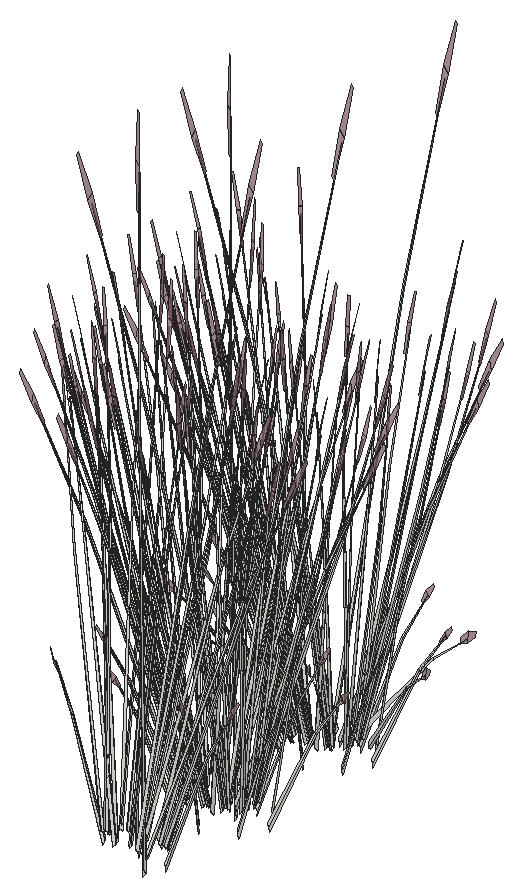
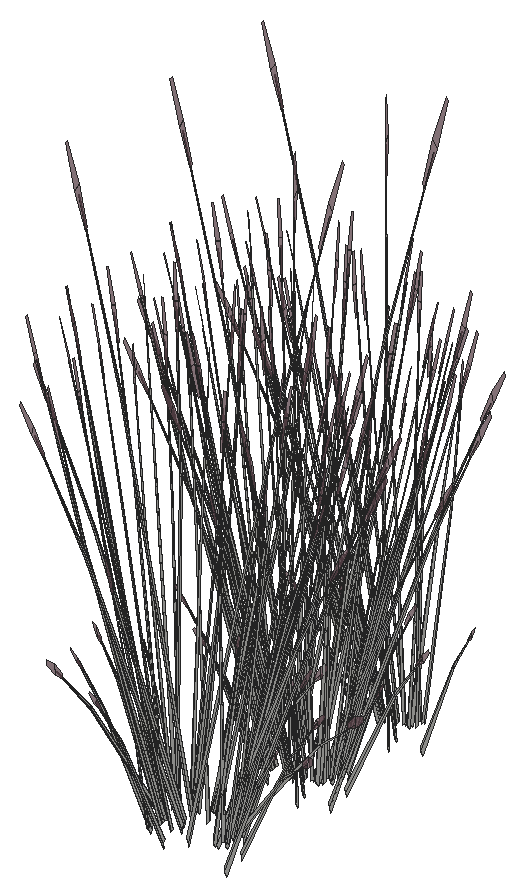
# SketchUp Ruby script. Lengths in inches.
U = 1.inch
M = Sketchup.active_model
def pt(a) = Geom::Point3d.new(a.map { |v| v * U })
def face(e, loops, mat)
  f = e.add_face(loops[0].map { |a| pt(a) })
  loops[1..].each { |l| e.add_face(l.map { |a| pt(a) }).erase! }
  f.material = f.back_material = mat if mat
  f
end
# faces: each face lists its corners as indices into pts; further lists are holes
def faces(e, pts, list, mat = nil) = list.each { |f| face(e, (f[0].is_a?(Array) ? f : [f]).map { |l| l.map { |i| pts[i] } }, mat) }
# xy, xz, yz: faces in a plane at the given z, y or x. An outline is a flat list of corners, or four numbers for a rectangle; further outlines are holes
def ring(l) = l.size == 4 ? [[l[0], l[1]], [l[2], l[1]], [l[2], l[3]], [l[0], l[3]]] : l.each_slice(2).to_a
def flat(e, list, mat, &to3) = list.each { |f| face(e, (f[0].is_a?(Array) ? f : [f]).map { |l| ring(l).map { |u, v| to3.(u, v) } }, mat) }
def xy(e, z, list, mat = nil) = flat(e, list, mat) { |x, y| [x, y, z] }
def xz(e, y, list, mat = nil) = flat(e, list, mat) { |x, z| [x, y, z] }
def yz(e, x, list, mat = nil) = flat(e, list, mat) { |y, z| [x, y, z] }
def lines(e, pts, list) = list.each { |a, b| e.add_line(pt(pts[a]), pt(pts[b])) }
# prism: a flat outline (further loops are holes) pulled along v
def prism(e, loops, v, mat = nil)
  f = face(e, loops, mat); d = Geom::Vector3d.new(v.map { |x| x * U })
  f.pushpull(f.normal.samedirection?(d) ? d.length : -d.length)
end
def box(e, o, s, mat = nil) = prism(e, [[o, [o[0] + s[0], o[1], o[2]], [o[0] + s[0], o[1] + s[1], o[2]], [o[0], o[1] + s[1], o[2]]]], [0, 0, s[2]], mat)
def at(x, y, z, deg = 0) = Geom::Transformation.translation(pt([x, y, z])) * Geom::Transformation.rotation(ORIGIN, Z_AXIS, deg.degrees)
def axes(o, x, y, z) = Geom::Transformation.new([*x, 0, *y, 0, *z, 0, *pt(o).to_a, 1])
def part(name) = M.definitions.add(name)
# library, detail: a bought-in or finely detailed component or shape, given as its bounding box
def library(name, o, s) = part(name).tap { |d| box(d.entities, o, s) }
def detail(e, o, s) = box(e.add_group.entities, o, s)
def put(e, d, t, mat = nil) = e.add_instance(d, t).tap { |i| i.material = mat if mat }
def group(e, t, mat = nil) = e.add_group.tap { |g| g.transformation = t; g.material = mat if mat }.entities
root = M.entities
M.materials.add("LightPink_Translucent").color = [144, 107, 117]
M.materials["LightPink_Translucent"].alpha = 0.75
c1 = part("blade")
p = [[2.15,0.21,22],[0,0.17,0],[0.09,0.45,0],[2.18,0.31,22],[2.29,0.31,22],[0.38,0.45,0],
  [2.48,0.24,33],[2.49,0.24,33],[2.48,0.22,33]]
faces(c1.entities,p,[[0,1,2,3],[4,5,2,3],[6,3,4,7],[8,0,3,6]])
c2 = part("seeds")
p = [[0.3,-0.1,1.38],[-0.01,-0.03,1.59],[-0.01,-0.03,0.03],[0.14,-0.07,-0.07],[0.29,-0.03,3],[0.15,0.01,3.11]]
faces(c2.entities,p,[[0,1,2,3],[1,0,4,5]],"LightPink_Translucent")
c3 = part("blade with seeds")
put(c3.entities,c1,at(0,0,0))
put(c3.entities,c2,axes([2.4,0.25,30.99],[1.5799,-0.05474,1.17369],[-0.12525,1.92788,0.29478],[-0.07173,-0.02425,1.56792]))
put(root,c3,axes([335.46,443.875,52.4],[0.50473,0.00941,-0.62776],[-0.0339,0.39618,0.07576],[0.21383,0.04181,0.88802]))
put(root,c3,axes([330.7,444.37,50.44],[0.21042,-0.1771,1.01491],[0.08303,0.28036,0.74569],[-0.15207,0.0502,0.22354]))
put(root,c3,axes([335.77,444.04,52],[0.28729,0.24465,-0.31292],[-0.32804,0.23159,0.40398],[0.16667,0.03524,0.77298]))
put(root,c3,axes([331.49,443.6,52],[-0.43951,0.05584,-0.31292],[-0.11606,-0.31924,0.40398],[-0.12595,0.08575,0.77298]))
put(root,c3,axes([334.73,443.41,51.43],[-0.18755,-0.06732,1.51428],[0.38813,-0.28243,0.12244],[0.24191,0.12741,0.64734]))
put(root,c3,axes([334.77,442.53,51.95],[-0.4363,-0.20303,1.22187],[0.46069,-0.31611,0.5272],[0.14077,0.1905,1.18105]))
put(root,c3,axes([331.625,443.38,52.45],[0.46706,0.21546,-0.10745],[-0.26908,0.31203,-0.59638],[-0.13196,0.10846,0.90619]))
put(root,c3,axes([335.43,444.18,50.44],[-0.28429,-0.11236,1.01491],[0.36709,-0.11416,0.74569],[0.09901,0.0967,0.22354]))
put(root,c3,axes([334.43,444.5,52.45],[0.30087,-0.33447,-0.10745],[0.43572,0.19269,-0.59638],[0.15146,0.0945,0.90619]))
put(root,c3,axes([332.25,443.29,51.43],[0.12611,-0.12006,1.51428],[0.31843,0.32408,0.12244],[-0.2184,0.14759,0.64734]))
put(root,c3,axes([331.86,443.64,52.14],[0.12971,0.3568,-0.45151],[-0.49122,0.06241,-0.34973],[-0.14077,0.09583,0.86392]))
put(root,c3,axes([334.74,442.91,50.51],[-0.01379,-0.36791,1.24828],[0.62424,0.09537,0.52853],[-0.14764,0.20132,1.17828]))
put(root,c3,axes([334.79,444.33,52.14],[0.49824,-0.09289,-0.45151],[0.08716,0.35177,-0.34973],[0.13382,0.10081,0.86392]))
put(root,c3,axes([332.69,449.72,51.43],[0.11542,0.12546,1.51428],[-0.53333,0.10562,0.12244],[-0.12054,-0.19696,0.64734]))
put(root,c3,axes([334.11,449.8125,52.4],[-0.24099,-0.31773,-0.62776],[0.49607,-0.17707,0.07576],[-0.05635,-0.15352,0.88802]))
put(root,c3,axes([332.16,443.58,51.43],[0.09401,-0.13431,1.51428],[0.3944,0.27795,0.12244],[-0.17792,0.17323,0.64734]))
put(root,c3,axes([332.27,444.34,52],[-0.34164,0.20573,-0.31292],[-0.3234,-0.23491,0.40398],[-0.04921,0.11936,0.77298]))
put(root,c3,axes([333.25,444.51,52.45],[0.49409,-0.18193,-0.10745],[0.24281,0.32289,-0.59638],[0.06519,0.13607,0.90619]))
put(root,c3,axes([335.12,450.125,52.4],[0.01314,-0.36145,-0.62776],[0.55324,0.02428,0.07576],[0.05838,-0.15313,0.88802]))
put(root,c3,axes([332.48,445.14,50.44],[-0.01307,-0.23234,1.01491],[0.32652,0.16572,0.74569],[-0.06422,0.11074,0.22354]))
put(root,c3,axes([334.16,449.54,52],[0.15222,-0.30049,-0.31292],[0.44409,0.08764,0.40398],[-0.04072,-0.12098,0.77298]))
put(root,c3,axes([334.5,449.94,51.43],[-0.09401,0.13431,1.51428],[-0.3944,-0.27795,0.12244],[0.17792,-0.17323,0.64734]))
put(root,c3,axes([332.61,444.24,52.42],[0.36145,0.26255,-0.50118],[-0.38183,0.22994,-0.3882],[-0.055,0.1334,0.95895]))
put(root,c3,axes([333.93,449.75,52.14],[-0.49634,-0.09796,-0.45151],[0.17013,-0.33585,-0.34973],[-0.04551,-0.13522,0.86392]))
put(root,c3,axes([334.24,448.91,50.44],[0.06477,0.22786,1.01491],[-0.35932,-0.1262,0.74569],[0.03867,-0.11667,0.22354]))
put(root,c3,axes([333.68,444.5,52.14],[0.49634,0.09796,-0.45151],[-0.17013,0.33585,-0.34973],[0.04551,0.13522,0.86392]))
put(root,c3,axes([335.01,450,52.14],[-0.36145,-0.26255,-0.45151],[0.38183,-0.22994,-0.34973],[0.055,-0.1334,0.86392]))
put(root,c3,axes([333.96,443.8,51.43],[-0.11542,-0.12546,1.51428],[0.53333,-0.10562,0.12244],[0.12054,0.19696,0.64734]))
put(root,c3,axes([333.45,444.7,52],[-0.15222,0.30049,-0.31292],[-0.44409,-0.08764,0.40398],[0.04072,0.12098,0.77298]))
put(root,c3,axes([332.49,444.12,52.72],[-0.01314,0.36145,-0.69681],[-0.55324,-0.02428,0.08409],[-0.05838,0.15313,0.9857]))
put(root,c3,axes([334.36,449.73,52.45],[-0.49409,0.18193,-0.10745],[-0.24281,-0.32289,-0.59638],[-0.06519,-0.13607,0.90619]))
put(root,c3,axes([335.38,450.14,52.45],[-0.55492,-0.01936,-0.10745],[0.01517,-0.36657,-0.59638],[0.03855,-0.14118,0.90619]))
put(root,c3,axes([335.35,449.91,52],[0.34164,-0.20573,-0.31292],[0.3234,0.23491,0.40398],[0.04921,-0.11936,0.77298]))
put(root,c3,axes([332.39,449.18,50.44],[0.26338,0.136,1.01491],[-0.38358,0.08175,0.74569],[-0.08207,-0.10452,0.22354]))
put(root,c3,axes([333.03,449.9,52.4],[-0.43054,-0.18887,-0.62776],[0.30598,-0.33097,0.07576],[-0.15599,-0.11277,0.88802]))
put(root,c3,axes([333.02,443.87,51.43],[-0.01236,-0.14998,1.51428],[0.53562,0.09949,0.12244],[-0.03313,0.21373,0.64734]))
put(root,c3,axes([332.88,449.65,52],[-0.07798,-0.31474,-0.31292],[0.44579,-0.08311,0.40398],[-0.11974,-0.09019,0.77298]))
put(root,c3,axes([333.5,444.43,52.4],[0.24099,0.31773,-0.62776],[-0.49607,0.17707,0.07576],[0.05635,0.15352,0.88802]))
put(root,c3,axes([331.92,450.11,51.43],[0.18755,0.06732,1.51428],[-0.38813,0.28243,0.12244],[-0.24191,-0.12741,0.64734]))
put(root,c3,axes([332.83,449.91,52.14],[-0.49824,0.09289,-0.45151],[-0.08716,-0.35177,-0.34973],[-0.13382,-0.10081,0.86392]))
put(root,c3,axes([332.31,444.63,50.97],[0.01109,-0.20172,1.3638],[0.49896,0.10655,0.18846],[-0.04323,0.21498,0.64398]))
put(root,c3,axes([335.77,450.75,52.4],[0.26374,-0.30832,-0.62776],[0.46217,0.21911,0.07576],[0.15748,-0.11171,0.88802]))
put(root,c3,axes([335.76,450.61,52.14],[-0.12971,-0.3568,-0.45151],[0.49122,-0.06241,-0.34973],[0.14077,-0.09583,0.86392]))
put(root,c3,axes([335.99,450.86,52.45],[-0.46706,-0.21546,-0.10745],[0.26908,-0.31203,-0.59638],[0.13196,-0.10846,0.90619]))
put(root,c3,axes([334.06,452.04,50.9375],[0.43633,0.15757,1.33654],[-0.42745,0.33945,0.52853],[-0.19146,-0.20119,1.12046]))
put(root,c3,axes([336.36,449.9,50.44],[-0.16818,0.19891,1.01491],[-0.14456,-0.26725,0.74569],[0.1389,-0.06697,0.22354]))
put(root,c3,axes([336.12,450.65,52],[0.43951,-0.05584,-0.31292],[0.11606,0.31924,0.40398],[0.12595,-0.08575,0.77298]))
put(root,c3,axes([331.85,450.21,52],[-0.28729,-0.24465,-0.31292],[0.32804,-0.23159,0.40398],[-0.16667,-0.03524,0.77298]))
put(root,c3,axes([332.15,450.37,52.4],[-0.50473,-0.00941,-0.62776],[0.0339,-0.39618,0.07576],[-0.21383,-0.04181,0.88802]))
put(root,c3,axes([331.98,450.45,52.14],[-0.36663,0.25884,-0.45151],[-0.32109,-0.27343,-0.34973],[-0.18628,-0.03938,0.86392]))
put(root,c3,axes([331.16,450.79,50.44],[0.32236,-0.02796,1.01491],[-0.20448,0.24636,0.74569],[-0.1593,-0.03696,0.22354]))
put(root,c3,axes([332.18,450.18,52.45],[-0.02704,0.39739,-0.10745],[-0.51189,-0.01086,-0.59638],[-0.19715,-0.0276,0.90619]))
put(root,c3,axes([336.01,451.7,52.45],[-0.25405,-0.35383,-0.10745],[0.45089,-0.17388,-0.59638],[0.19001,-0.04668,0.90619]))
put(root,c3,axes([335.98,451.4,52.14],[0.13679,-0.35544,-0.45151],[0.46898,0.12183,-0.34973],[0.18882,-0.03259,0.86392]))
put(root,c3,axes([331.52,450.73,51.43],[0.20943,-0.00885,1.51428],[-0.13893,0.38357,0.12244],[-0.29846,-0.02372,0.64734]))
put(root,c3,axes([335.9,451.53,52.4],[0.44368,-0.17257,-0.62776],[0.24726,0.35524,0.07576],[0.21437,-0.04035,0.88802]))
put(root,c3,axes([336.27,451.5625,52],[0.41962,0.10901,-0.31292],[-0.12239,0.31802,0.40398],[0.16894,-0.02916,0.77298]))
put(root,c3,axes([331.34,451.06,52],[-0.41962,-0.10901,-0.31292],[0.12239,-0.31802,0.40398],[-0.16894,0.02916,0.77298]))
put(root,c3,axes([335.13,451.17,51.43],[-0.20943,0.00885,1.51428],[0.13893,-0.38357,0.12244],[0.29846,0.02372,0.64734]))
put(root,c3,axes([332.62,451,50.95],[0.14352,-0.05653,1.56454],[0.04949,0.39467,0.12244],[-0.31087,0.05237,0.55918]))
put(root,c3,axes([337.16,451.63,50.44],[-0.31197,0.06451,1.01491],[0.14684,-0.26661,0.74569],[0.1655,0.01824,0.22354]))
put(root,c3,axes([331.63,451.22,52.14],[-0.13679,0.35544,-0.45151],[-0.46898,-0.12183,-0.34973],[-0.18882,0.03259,0.86392]))
put(root,c3,axes([331.61,450.91,52.45],[0.25405,0.35383,-0.10745],[-0.45089,0.17388,-0.59638],[-0.19001,0.04668,0.90619]))
put(root,c3,axes([336.62,452.45,51.47],[-0.09664,-0.32847,-0.03085],[0.45676,-0.07551,-0.13989],[0.09538,0.02082,0.4614]))
put(root,c3,axes([335.4375,452.44,52.45],[0.02704,-0.39739,-0.10745],[0.51189,0.01086,-0.59638],[0.19715,0.0276,0.90619]))
put(root,c3,axes([331.61,451.4,51.43],[0.17519,-0.08265,1.51428],[0.14749,0.38193,0.12244],[-0.27504,0.08632,0.64734]))
put(root,c3,axes([335.46,452.25,52.4],[0.50473,0.00941,-0.62776],[-0.0339,0.39618,0.07576],[0.21383,0.04181,0.88802]))
put(root,c3,axes([330.7,452.74,50.44],[0.21042,-0.1771,1.01491],[0.08303,0.28036,0.74569],[-0.15207,0.0502,0.22354]))
put(root,c3,axes([335.77,452.41,52],[0.28729,0.24465,-0.31292],[-0.32804,0.23159,0.40398],[0.16667,0.03524,0.77298]))
put(root,c3,axes([331.49,451.97,52],[-0.43951,0.05584,-0.31292],[-0.11606,-0.31924,0.40398],[-0.12595,0.08575,0.77298]))
put(root,c3,axes([334.73,451.79,51.43],[-0.18755,-0.06732,1.51428],[0.38813,-0.28243,0.12244],[0.24191,0.12741,0.64734]))
put(root,c3,axes([334.77,450.9,51.95],[-0.4363,-0.20303,1.22187],[0.46069,-0.31611,0.5272],[0.14077,0.1905,1.18105]))
put(root,c3,axes([331.625,451.76,52.45],[0.46706,0.21546,-0.10745],[-0.26908,0.31203,-0.59638],[-0.13196,0.10846,0.90619]))
put(root,c3,axes([335.43,452.55,50.44],[-0.28429,-0.11236,1.01491],[0.36709,-0.11416,0.74569],[0.09901,0.0967,0.22354]))
put(root,c3,axes([334.43,452.87,52.45],[0.30087,-0.33447,-0.10745],[0.43572,0.19269,-0.59638],[0.15146,0.0945,0.90619]))
put(root,c3,axes([332.25,451.66,51.43],[0.12611,-0.12006,1.51428],[0.31843,0.32408,0.12244],[-0.2184,0.14759,0.64734]))
put(root,c3,axes([331.86,452.01,52.14],[0.12971,0.3568,-0.45151],[-0.49122,0.06241,-0.34973],[-0.14077,0.09583,0.86392]))
put(root,c3,axes([334.74,451.29,50.51],[-0.01379,-0.36791,1.24828],[0.62424,0.09537,0.52853],[-0.14764,0.20132,1.17828]))
put(root,c3,axes([334.79,452.71,52.14],[0.49824,-0.09289,-0.45151],[0.08716,0.35177,-0.34973],[0.13382,0.10081,0.86392]))
put(root,c3,axes([332.16,451.96,51.43],[0.09401,-0.13431,1.51428],[0.3944,0.27795,0.12244],[-0.17792,0.17323,0.64734]))
put(root,c3,axes([332.27,452.71,52],[-0.34164,0.20573,-0.31292],[-0.3234,-0.23491,0.40398],[-0.04921,0.11936,0.77298]))
put(root,c3,axes([333.25,452.89,52.45],[0.49409,-0.18193,-0.10745],[0.24281,0.32289,-0.59638],[0.06519,0.13607,0.90619]))
put(root,c3,axes([332.48,453.51,50.44],[-0.01307,-0.23234,1.01491],[0.32652,0.16572,0.74569],[-0.06422,0.11074,0.22354]))
put(root,c3,axes([332.61,452.62,52.42],[0.36145,0.26255,-0.50118],[-0.38183,0.22994,-0.3882],[-0.055,0.1334,0.95895]))
put(root,c3,axes([333.68,452.87,52.14],[0.49634,0.09796,-0.45151],[-0.17013,0.33585,-0.34973],[0.04551,0.13522,0.86392]))
put(root,c3,axes([333.96,452.18,51.43],[-0.11542,-0.12546,1.51428],[0.53333,-0.10562,0.12244],[0.12054,0.19696,0.64734]))
put(root,c3,axes([333.45,453.08,52],[-0.15222,0.30049,-0.31292],[-0.44409,-0.08764,0.40398],[0.04072,0.12098,0.77298]))
put(root,c3,axes([332.49,452.5,52.72],[-0.01314,0.36145,-0.69681],[-0.55324,-0.02428,0.08409],[-0.05838,0.15313,0.9857]))
put(root,c3,axes([332.69,459.23,51.43],[0.11542,0.12546,1.51428],[-0.53333,0.10562,0.12244],[-0.12054,-0.19696,0.64734]))
put(root,c3,axes([333.02,452.24,51.43],[-0.01236,-0.14998,1.51428],[0.53562,0.09949,0.12244],[-0.03313,0.21373,0.64734]))
put(root,c3,axes([333.57,458.4,52.17],[-0.07723,-0.05479,1.54581],[-0.51538,0.03473,-0.24447],[-0.08225,-0.13104,0.12397]))
put(root,c3,axes([334.11,459.33,52.4],[-0.24099,-0.31773,-0.62776],[0.49607,-0.17707,0.07576],[-0.05635,-0.15352,0.88802]))
put(root,c3,axes([333.5,452.81,52.4],[0.24099,0.31773,-0.62776],[-0.49607,0.17707,0.07576],[0.05635,0.15352,0.88802]))
put(root,c3,axes([335.12,459.64,52.4],[0.01314,-0.36145,-0.62776],[0.55324,0.02428,0.07576],[0.05838,-0.15313,0.88802]))
put(root,c3,axes([335.89,459.07,52.17],[-0.00487,-0.07777,1.54581],[-0.41166,-0.22476,-0.24447],[0.06364,-0.13625,0.12397]))
put(root,c3,axes([334.16,459.06,52],[0.15222,-0.30049,-0.31292],[0.44409,0.08764,0.40398],[-0.04072,-0.12098,0.77298]))
put(root,c3,axes([334.5,459.46,51.43],[-0.09401,0.13431,1.51428],[-0.3944,-0.27795,0.12244],[0.17792,-0.17323,0.64734]))
put(root,c3,axes([333.93,459.26,52.14],[-0.49634,-0.09796,-0.45151],[0.17013,-0.33585,-0.34973],[-0.04551,-0.13522,0.86392]))
put(root,c3,axes([334.24,458.42,50.44],[0.06477,0.22786,1.01491],[-0.35932,-0.1262,0.74569],[0.03867,-0.11667,0.22354]))
put(root,c3,axes([332.31,453,50.97],[0.01109,-0.20172,1.3638],[0.49896,0.10655,0.18846],[-0.04323,0.21498,0.64398]))
put(root,c3,axes([335.01,459.52,52.14],[-0.36145,-0.26255,-0.45151],[0.38183,-0.22994,-0.34973],[0.055,-0.1334,0.86392]))
put(root,c3,axes([334.36,459.25,52.45],[-0.49409,0.18193,-0.10745],[-0.24281,-0.32289,-0.59638],[-0.06519,-0.13607,0.90619]))
put(root,c3,axes([335.38,459.66,52.45],[-0.55492,-0.01936,-0.10745],[0.01517,-0.36657,-0.59638],[0.03855,-0.14118,0.90619]))
put(root,c3,axes([335.35,459.42,52],[0.34164,-0.20573,-0.31292],[0.3234,0.23491,0.40398],[0.04921,-0.11936,0.77298]))
put(root,c3,axes([332.39,458.7,50.44],[0.26338,0.136,1.01491],[-0.38358,0.08175,0.74569],[-0.08207,-0.10452,0.22354]))
put(root,c3,axes([333.03,459.42,52.4],[-0.43054,-0.18887,-0.62776],[0.30598,-0.33097,0.07576],[-0.15599,-0.11277,0.88802]))
put(root,c3,axes([332.88,459.17,52],[-0.07798,-0.31474,-0.31292],[0.44579,-0.08311,0.40398],[-0.11974,-0.09019,0.77298]))
put(root,c3,axes([331.92,459.625,51.43],[0.18755,0.06732,1.51428],[-0.38813,0.28243,0.12244],[-0.24191,-0.12741,0.64734]))
put(root,c3,axes([332.83,459.43,52.14],[-0.49824,0.09289,-0.45151],[-0.08716,-0.35177,-0.34973],[-0.13382,-0.10081,0.86392]))
put(root,c3,axes([335.77,460.27,52.4],[0.26374,-0.30832,-0.62776],[0.46217,0.21911,0.07576],[0.15748,-0.11171,0.88802]))
put(root,c3,axes([335.76,460.125,52.14],[-0.12971,-0.3568,-0.45151],[0.49122,-0.06241,-0.34973],[0.14077,-0.09583,0.86392]))
put(root,c3,axes([331.88,459.01,52.17],[-0.10864,-0.00276,1.54581],[-0.34587,0.27582,-0.24447],[-0.18454,-0.05636,0.12397]))
put(root,c3,axes([335.99,460.38,52.45],[-0.46706,-0.21546,-0.10745],[0.26908,-0.31203,-0.59638],[0.13196,-0.10846,0.90619]))
put(root,c3,axes([334.06,461.55,50.9375],[0.43633,0.15757,1.33654],[-0.42745,0.33945,0.52853],[-0.19146,-0.20119,1.12046]))
put(root,c3,axes([336.36,459.41,50.44],[-0.16818,0.19891,1.01491],[-0.14456,-0.26725,0.74569],[0.1389,-0.06697,0.22354]))
put(root,c3,axes([336.12,460.16,52],[0.43951,-0.05584,-0.31292],[0.11606,0.31924,0.40398],[0.12595,-0.08575,0.77298]))
put(root,c3,axes([331.85,459.72,52],[-0.28729,-0.24465,-0.31292],[0.32804,-0.23159,0.40398],[-0.16667,-0.03524,0.77298]))
put(root,c3,axes([332.15,459.89,52.4],[-0.50473,-0.00941,-0.62776],[0.0339,-0.39618,0.07576],[-0.21383,-0.04181,0.88802]))
put(root,c3,axes([337.39,460.66,52.17],[0.07006,-0.05952,1.54581],[-0.08968,-0.3651,-0.24447],[0.1758,-0.06922,0.12397]))
put(root,c3,axes([331.98,459.97,52.14],[-0.36663,0.25884,-0.45151],[-0.32109,-0.27343,-0.34973],[-0.18628,-0.03938,0.86392]))
put(root,c3,axes([331.16,460.31,50.44],[0.32236,-0.02796,1.01491],[-0.20448,0.24636,0.74569],[-0.1593,-0.03696,0.22354]))
put(root,c3,axes([332.18,459.69,52.45],[-0.02704,0.39739,-0.10745],[-0.51189,-0.01086,-0.59638],[-0.19715,-0.0276,0.90619]))
put(root,c3,axes([336.01,461.22,52.45],[-0.25405,-0.35383,-0.10745],[0.45089,-0.17388,-0.59638],[0.19001,-0.04668,0.90619]))
put(root,c3,axes([335.98,460.92,52.14],[0.13679,-0.35544,-0.45151],[0.46898,0.12183,-0.34973],[0.18882,-0.03259,0.86392]))
put(root,c3,axes([331.52,460.24,51.43],[0.20943,-0.00885,1.51428],[-0.13893,0.38357,0.12244],[-0.29846,-0.02372,0.64734]))
put(root,c3,axes([335.9,461.04,52.4],[0.44368,-0.17257,-0.62776],[0.24726,0.35524,0.07576],[0.21437,-0.04035,0.88802]))
put(root,c3,axes([336.27,461.08,52],[0.41962,0.10901,-0.31292],[-0.12239,0.31802,0.40398],[0.16894,-0.02916,0.77298]))
put(root,c3,axes([331.34,460.57,52],[-0.41962,-0.10901,-0.31292],[0.12239,-0.31802,0.40398],[-0.16894,0.02916,0.77298]))
put(root,c3,axes([335.13,460.68,51.43],[-0.20943,0.00885,1.51428],[0.13893,-0.38357,0.12244],[0.29846,0.02372,0.64734]))
put(root,c3,axes([332.62,460.52,50.95],[0.14352,-0.05653,1.56454],[0.04949,0.39467,0.12244],[-0.31087,0.05237,0.55918]))
put(root,c3,axes([337.16,461.14,50.44],[-0.31197,0.06451,1.01491],[0.14684,-0.26661,0.74569],[0.1655,0.01824,0.22354]))
put(root,c3,axes([331.08,460.78,52.17],[-0.08245,0.05073,1.54581],[0.00701,0.37067,-0.24447],[-0.18899,0.0482,0.12397]))
put(root,c3,axes([331.63,460.73,52.14],[-0.13679,0.35544,-0.45151],[-0.46898,-0.12183,-0.34973],[-0.18882,0.03259,0.86392]))
put(root,c3,axes([331.61,460.43,52.45],[0.25405,0.35383,-0.10745],[-0.45089,0.17388,-0.59638],[-0.19001,0.04668,0.90619]))
put(root,c3,axes([336.62,461.96,51.47],[-0.09664,-0.32847,-0.03085],[0.45676,-0.07551,-0.13989],[0.09538,0.02082,0.4614]))
put(root,c3,axes([335.4375,461.95,52.45],[0.02704,-0.39739,-0.10745],[0.51189,0.01086,-0.59638],[0.19715,0.0276,0.90619]))
put(root,c3,axes([335.88,461.72,52.17],[0.10831,-0.00661,1.54581],[0.29709,-0.30358,-0.24447],[0.19266,0.04007,0.12397]))
put(root,c3,axes([331.61,460.92,51.43],[0.17519,-0.08265,1.51428],[0.14749,0.38193,0.12244],[-0.27504,0.08632,0.64734]))
put(root,c3,axes([335.46,461.76,52.4],[0.50473,0.00941,-0.62776],[-0.0339,0.39618,0.07576],[0.21383,0.04181,0.88802]))
put(root,c3,axes([330.7,462.25,50.44],[0.21042,-0.1771,1.01491],[0.08303,0.28036,0.74569],[-0.15207,0.0502,0.22354]))
put(root,c3,axes([335.77,461.93,52],[0.28729,0.24465,-0.31292],[-0.32804,0.23159,0.40398],[0.16667,0.03524,0.77298]))
put(root,c3,axes([331.49,461.49,52],[-0.43951,0.05584,-0.31292],[-0.11606,-0.31924,0.40398],[-0.12595,0.08575,0.77298]))
put(root,c3,axes([334.73,461.3,51.43],[-0.18755,-0.06732,1.51428],[0.38813,-0.28243,0.12244],[0.24191,0.12741,0.64734]))
put(root,c3,axes([334.77,460.41,51.95],[-0.4363,-0.20303,1.22187],[0.46069,-0.31611,0.5272],[0.14077,0.1905,1.18105]))
put(root,c3,axes([331.625,461.27,52.45],[0.46706,0.21546,-0.10745],[-0.26908,0.31203,-0.59638],[-0.13196,0.10846,0.90619]))
put(root,c3,axes([335.43,462.07,50.44],[-0.28429,-0.11236,1.01491],[0.36709,-0.11416,0.74569],[0.09901,0.0967,0.22354]))
put(root,c3,axes([334.43,462.39,52.45],[0.30087,-0.33447,-0.10745],[0.43572,0.19269,-0.59638],[0.15146,0.0945,0.90619]))
put(root,c3,axes([332.25,461.17,51.43],[0.12611,-0.12006,1.51428],[0.31843,0.32408,0.12244],[-0.2184,0.14759,0.64734]))
